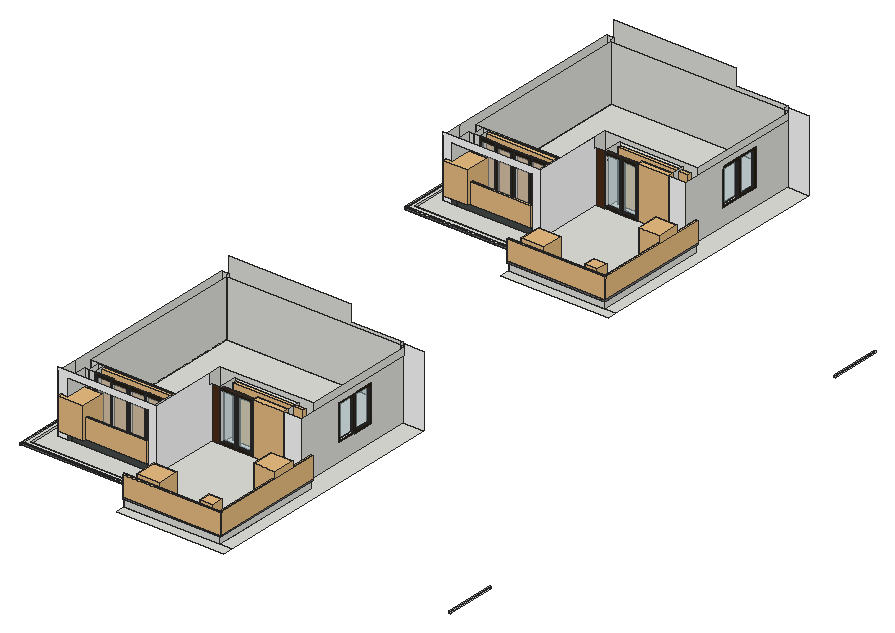
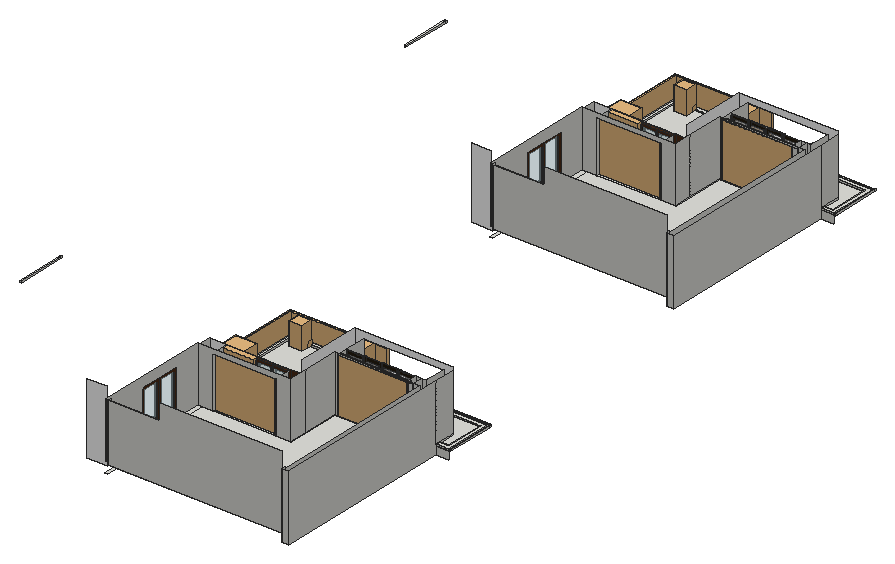
# SketchUp Ruby script. Lengths in inches.
U = 1.inch
M = Sketchup.active_model
def pt(a) = Geom::Point3d.new(a.map { |v| v * U })
def face(e, loops, mat)
  f = e.add_face(loops[0].map { |a| pt(a) })
  loops[1..].each { |l| e.add_face(l.map { |a| pt(a) }).erase! }
  f.material = f.back_material = mat if mat
  f
end
# faces: each face lists its corners as indices into pts; further lists are holes
def faces(e, pts, list, mat = nil) = list.each { |f| face(e, (f[0].is_a?(Array) ? f : [f]).map { |l| l.map { |i| pts[i] } }, mat) }
# xy, xz, yz: faces in a plane at the given z, y or x. An outline is a flat list of corners, or four numbers for a rectangle; further outlines are holes
def ring(l) = l.size == 4 ? [[l[0], l[1]], [l[2], l[1]], [l[2], l[3]], [l[0], l[3]]] : l.each_slice(2).to_a
def flat(e, list, mat, &to3) = list.each { |f| face(e, (f[0].is_a?(Array) ? f : [f]).map { |l| ring(l).map { |u, v| to3.(u, v) } }, mat) }
def xy(e, z, list, mat = nil) = flat(e, list, mat) { |x, y| [x, y, z] }
def xz(e, y, list, mat = nil) = flat(e, list, mat) { |x, z| [x, y, z] }
def yz(e, x, list, mat = nil) = flat(e, list, mat) { |y, z| [x, y, z] }
def lines(e, pts, list) = list.each { |a, b| e.add_line(pt(pts[a]), pt(pts[b])) }
# prism: a flat outline (further loops are holes) pulled along v
def prism(e, loops, v, mat = nil)
  f = face(e, loops, mat); d = Geom::Vector3d.new(v.map { |x| x * U })
  f.pushpull(f.normal.samedirection?(d) ? d.length : -d.length)
end
def box(e, o, s, mat = nil) = prism(e, [[o, [o[0] + s[0], o[1], o[2]], [o[0] + s[0], o[1] + s[1], o[2]], [o[0], o[1] + s[1], o[2]]]], [0, 0, s[2]], mat)
def at(x, y, z, deg = 0) = Geom::Transformation.translation(pt([x, y, z])) * Geom::Transformation.rotation(ORIGIN, Z_AXIS, deg.degrees)
def axes(o, x, y, z) = Geom::Transformation.new([*x, 0, *y, 0, *z, 0, *pt(o).to_a, 1])
def part(name) = M.definitions.add(name)
# library, detail: a bought-in or finely detailed component or shape, given as its bounding box
def library(name, o, s) = part(name).tap { |d| box(d.entities, o, s) }
def detail(e, o, s) = box(e.add_group.entities, o, s)
def put(e, d, t, mat = nil) = e.add_instance(d, t).tap { |i| i.material = mat if mat }
def group(e, t, mat = nil) = e.add_group.tap { |g| g.transformation = t; g.material = mat if mat }.entities
root = M.entities
M.materials.add("[Color M00]").color = [255, 255, 255]
M.materials.add("[Color M05]").color = [114, 114, 114]
M.materials.add("[Slate]").color = [70, 76, 75]
M.materials.add("[Translucent Glass Gray]2").color = [201, 201, 201]
M.materials["[Translucent Glass Gray]2"].alpha = 0.5
M.materials.add("[Translucent Glass Safety]").color = [204, 235, 244]
M.materials["[Translucent Glass Safety]"].alpha = 0.5
M.materials.add("[Wood Veneer 01]").color = [76, 44, 23]
M.materials.add("oak swatch").color = [40, 31, 19]
c1 = library("plant (1)",[-35.72,-28.42,0],[66.31,67.39,84.38])
c2 = library("Glass Railing",[0,0,0],[139.5,4.76,42])
c3 = part("Group\#6")
box(c3.entities,[0,0,0],[1.77,4.72,80.31],"oak swatch")
c4 = part("Exterior Sliding Doors")
xy(c4.entities,0,[[1.77,33.07,3.54,70.87],[1.77,70.87,3.54,108.66]])
xy(c4.entities,0,[[0,0,1.77,33.07],[0,108.66,1.77,141.73]],"oak swatch")
xy(c4.entities,4.72,[[0,4.72,1.77,33.07],[1.77,37.8,3.54,66.14],[1.77,75.88,3.54,103.9375],[0,108.66,1.77,137.01]],"oak swatch")
xy(c4.entities,75.59,[[1.77,37.8,3.54,66.14],[1.77,75.88,3.54,103.9375]])
xy(c4.entities,75.59,[[0,4.72,1.77,33.07],[0,108.66,1.77,137.01]],"oak swatch")
xy(c4.entities,80.31,[[0,0,1.77,33.07],[1.77,33.07,3.54,70.87],[1.77,70.87,3.54,108.66],[0,108.66,1.77,141.73]],"oak swatch")
xz(c4.entities,0,[[0,0,1.77,80.31]],"oak swatch")
xz(c4.entities,4.72,[[0,4.72,1.77,75.59]],"oak swatch")
xz(c4.entities,33.07,[[0,0,1.77,4.72],[1.77,0,3.54,80.31],[0,75.59,1.77,80.31]],"oak swatch")
xz(c4.entities,37.8,[[1.77,4.72,3.54,75.59]])
xz(c4.entities,66.14,[[1.77,4.72,3.54,75.59]],"oak swatch")
xz(c4.entities,70.87,[[1.77,0,3.54,80.31]])
xz(c4.entities,75.88,[[1.77,4.72,3.54,75.59]])
xz(c4.entities,103.9375,[[1.77,4.72,3.54,75.59]],"oak swatch")
xz(c4.entities,108.66,[[1.77,4.72,3.54,75.59]])
xz(c4.entities,108.66,[[0,0,3.54,4.72],[0,75.59,3.54,80.31]],"oak swatch")
xz(c4.entities,137.01,[[0,4.72,1.77,75.59]],"oak swatch")
xz(c4.entities,141.73,[[0,0,1.77,80.31]],"oak swatch")
yz(c4.entities,0,[[0,0,33.07,0,33.07,4.72,4.72,4.72,4.72,75.59,33.07,75.59,33.07,80.31,0,80.31],[108.66,0,141.73,0,141.73,80.31,108.66,80.31,108.66,75.59,137.01,75.59,137.01,4.72,108.66,4.72]],"oak swatch")
yz(c4.entities,1.77,[[4.72,4.72,33.07,75.59],[37.8,4.72,66.14,75.59],[75.88,4.72,103.9375,75.59],[108.66,4.72,137.01,75.59]],"[Translucent Glass Gray]2")
yz(c4.entities,1.77,[[0,0,33.07,0,33.07,4.72,4.72,4.72,4.72,75.59,33.07,75.59,33.07,80.31,0,80.31],[[33.07,0,70.87,80.31],[37.8,4.72,66.14,75.59]],[[70.87,0,141.73,80.31],[108.66,4.72,137.01,75.59],[75.88,4.72,103.9375,75.59]]],"oak swatch")
yz(c4.entities,3.54,[[[33.07,0,70.87,80.31],[37.8,4.72,66.14,75.59]],[[70.87,0,108.66,80.31],[75.88,4.72,103.9375,75.59]]],"oak swatch")
put(c4.entities,c3,at(0,33.07,0))
put(c4.entities,c3,at(0,103.9375,0))
c5 = library("Curtains",[0,0,0],[121.73,8.19,117.22])
c6 = library("Plant",[0,0,0],[12.59,12.59,14.16])
c7 = part("Group\#4")
g1 = group(c7.entities,at(0,0,0))
xy(g1,0,[[0,0,6,48]],"[Wood Veneer 01]")
xy(g1,4,[[0,4,1.8125,44],[1.8125,4,6,44]])
xy(g1,80,[[0,4,1.8125,44],[1.8125,4,6,44]])
xy(g1,84,[[0,0,6,48]],"[Wood Veneer 01]")
xz(g1,0,[[0,0,6,84]],"[Wood Veneer 01]")
xz(g1,4,[[0,4,1.8125,80],[1.8125,4,6,80]])
xz(g1,44,[[0,4,1.8125,80],[1.8125,4,6,80]])
xz(g1,48,[[0,0,6,84]],"[Wood Veneer 01]")
yz(g1,0,[[[0,0,48,84],[4,4,44,80]]],"[Wood Veneer 01]")
yz(g1,1.8125,[[4,4,44,80]],"[Translucent Glass Safety]")
yz(g1,6,[[[0,0,48,84],[4,4,44,80]]],"oak swatch")
g2 = group(c7.entities,at(0,48,0),"oak swatch")
xy(g2,0,[[0,0,6,48]],"[Wood Veneer 01]")
xy(g2,4,[[0,4,1.8125,44],[1.8125,4,6,44]])
xy(g2,80,[[0,4,1.8125,44],[1.8125,4,6,44]])
xy(g2,84,[[0,0,6,48]],"[Wood Veneer 01]")
xz(g2,0,[[0,0,6,84]],"[Wood Veneer 01]")
xz(g2,4,[[0,4,1.8125,80],[1.8125,4,6,80]])
xz(g2,44,[[0,4,1.8125,80],[1.8125,4,6,80]])
xz(g2,48,[[0,0,6,84]],"[Wood Veneer 01]")
yz(g2,0,[[[0,0,48,84],[4,4,44,80]]],"[Wood Veneer 01]")
yz(g2,1.8125,[[4,4,44,80]],"[Translucent Glass Safety]")
yz(g2,6,[[[0,0,48,84],[4,4,44,80]]],"oak swatch")
c8 = library("Flora+17",[-57.52,158.6,-38.64],[66.99,62.88,77.28])
c9 = library("modern+door",[0,0,0],[59.06,11.8125,86.61])
c10 = library("plant1",[-367.84,-375.82,-125.45],[750.59,696.16,1346.74])
c11 = part("skp4FF")
put(c11.entities,c10,at(0,0,0))
xy(root,121.3125,[[491.71,481.81,715.11,502.24],[491.71,502.24,690.8,538.49],[690.8,502.24,715.11,502.24,715.11,1001.66,671.36,1001.66,671.36,738.06,690.8,738.06],[491.71,538.49,690.8,638.99],[279.74,638.99,279.74,1021.31,294.47,1021.31,294.47,662.52,312.05,662.52,312.05,638.99],
  [491.71,638.99,690.8,738.06],[312.05,648.22,312.05,662.52,471.68,662.52,471.68,776.62,481.36,776.62,481.36,648.22],[491.71,738.06,671.36,749.87],[655.66,813.85,662.14,1021.31],[491.71,1481.16,715.11,1501.6],
  [491.71,1501.6,690.8,1537.85],[690.8,1501.6,715.11,1501.6,715.11,2001.02,671.36,2001.02,671.36,1737.41,690.8,1737.41],[491.71,1537.85,690.8,1638.35],[279.74,1638.35,279.74,2020.66,294.47,2020.66,294.47,1661.875,312.05,1661.875,312.05,1638.35],[491.71,1638.35,690.8,1737.41],
  [312.05,1647.57,312.05,1661.875,471.68,1661.875,471.68,1775.97,481.36,1775.97,481.36,1647.57],[491.71,1737.41,671.36,1749.22],[655.66,1813.21,662.14,2020.66]])
xy(root,138.1875,[[491.71,497.56,690.8,502.24],[690.8,497.56,695.49,502.24],[491.71,502.24,491.71,538.49,252.74,538.49,252.74,638.99,279.74,638.99,279.74,630.62,260.99,630.62,260.99,547.12,498.05,547.12,498.05,510.06,684.49,510.06,684.49,724.25,671.36,724.25,671.36,738.06,690.8,738.06,690.8,502.24],[690.8,502.24,695.49,738.06],[498.05,510.06,684.49,510.06,684.49,724.25,671.36,724.25,671.36,738.06,484.3,738.06,484.3,595.06,279.74,595.06,279.74,630.62,260.99,630.62,260.99,547.12,498.05,547.12],
  [249.43,533.81,252.74,538.49],[252.74,533.81,491.71,538.49],[249.43,538.49,252.55,638.99],[252.55,538.49,252.74,638.99],[1142.02,538.49,1145.14,638.99],
  [279.74,595.06,308.96,595.06,308.96,606.41,299.58,606.41,299.58,638.99,279.74,638.99],[466.14,595.06,484.3,638.99],[299.58,606.41,466.14,638.99],[308.96,638.99,321.33,662.52],[321.33,638.99,466.14,662.52],
  [294.47,662.52,471.68,662.52,471.68,776.62,655.66,776.62,655.66,1014.93,294.47,1014.93],[502.34,738.06,634.66,776.62],[655.66,776.62,665.66,1014.93],[294.47,1014.93,655.66,1021.31],[491.71,1496.91,690.8,1501.6],
  [690.8,1496.91,695.49,1501.6],[491.71,1501.6,491.71,1537.85,252.74,1537.85,252.74,1638.35,279.74,1638.35,279.74,1629.97,260.99,1629.97,260.99,1546.47,498.05,1546.47,498.05,1509.41,684.49,1509.41,684.49,1723.61,671.36,1723.61,671.36,1737.41,690.8,1737.41,690.8,1501.6],[690.8,1501.6,695.49,1737.41],[498.05,1509.41,684.49,1509.41,684.49,1723.61,671.36,1723.61,671.36,1737.41,484.3,1737.41,484.3,1594.41,279.74,1594.41,279.74,1629.97,260.99,1629.97,260.99,1546.47,498.05,1546.47],[249.43,1533.16,252.74,1537.85],
  [252.74,1533.16,491.71,1537.85],[1142.02,1533.16,1145.33,1537.85],[249.43,1537.85,252.55,1638.35],[252.55,1537.85,252.74,1638.35],[1142.02,1537.85,1145.14,1638.35],
  [279.74,1594.41,308.96,1594.41,308.96,1605.76,299.58,1605.76,299.58,1638.35,279.74,1638.35],[466.14,1594.41,484.3,1638.35],[299.58,1605.76,466.14,1638.35],[308.96,1638.35,321.33,1661.875],[321.33,1638.35,466.14,1661.875],
  [294.47,1661.875,471.68,1661.875,471.68,1775.97,655.66,1775.97,655.66,2014.29,294.47,2014.29],[502.34,1737.41,634.66,1775.97],[655.66,1775.97,665.66,2014.29],[294.47,2014.29,655.66,2020.66]])
xy(root,141.4375,[[491.71,497.56,695.49,497.56,695.49,738.06,690.8,738.06,690.8,502.24,491.71,502.24],[491.71,502.24,690.8,502.24,690.8,738.06,671.36,738.06,671.36,724.25,684.49,724.25,684.49,510.06,498.05,510.06,498.05,547.12,260.99,547.12,260.99,630.62,279.74,630.62,279.74,638.99,252.74,638.99,252.74,538.49,491.71,538.49],[249.43,533.81,252.74,538.49],[252.74,533.81,491.71,538.49],[249.43,538.49,252.55,638.99],
  [252.55,538.49,252.74,638.99],[1142.02,538.49,1145.14,638.99],[491.71,1496.91,695.49,1496.91,695.49,1737.41,690.8,1737.41,690.8,1501.6,491.71,1501.6],[491.71,1501.6,690.8,1501.6,690.8,1737.41,671.36,1737.41,671.36,1723.61,684.49,1723.61,684.49,1509.41,498.05,1509.41,498.05,1546.47,260.99,1546.47,260.99,1629.97,279.74,1629.97,279.74,1638.35,252.74,1638.35,252.74,1537.85,491.71,1537.85],[249.43,1533.16,252.74,1537.85],
  [252.74,1533.16,491.71,1537.85],[249.43,1537.85,252.55,1638.35],[252.55,1537.85,252.74,1638.35],[1142.02,1537.85,1145.14,1638.35]])
xy(root,152,[[299.58,595.06,308.96,606.41],[308.96,595.06,466.14,606.41],[299.58,1594.41,308.96,1605.76],[308.96,1594.41,466.14,1605.76]],"[Slate]")
xy(root,155.89,[[665.66,833.57,671.36,919.13],[665.66,1832.92,671.36,1918.48]])
xz(root,497.56,[[491.71,138.1875,695.49,141.4375]],"[Color M05]")
xz(root,502.24,[[491.71,121.3125,690.8,138.1875],[491.71,138.1875,690.8,141.4375]])
xz(root,510.06,[[498.05,138.1875,684.49,141.4375]])
xz(root,533.81,[[249.43,138.1875,252.74,141.4375],[1142.02,138.1875,1145.33,141.4375]])
xz(root,533.81,[[252.74,138.1875,491.71,141.4375]],"[Color M05]")
xz(root,538.49,[[249.43,138.1875,252.55,141.4375],[252.55,138.1875,252.74,141.4375],[252.74,138.1875,491.71,141.4375],[1142.02,138.1875,1145.14,141.4375]])
xz(root,547.12,[[260.99,138.1875,498.05,141.4375]])
xz(root,595.06,[[279.74,138.1875,299.58,138.1875,299.58,252.5,466.14,252.5,466.14,138.1875,484.3,138.1875,484.3,265.6875,279.74,265.6875]],"[Color M00]")
xz(root,595.06,[[299.58,138.1875,308.96,152],[308.96,138.1875,466.14,152]],"[Slate]")
xz(root,606.41,[[299.58,138.1875,308.96,152],[308.96,138.1875,466.14,152]])
xz(root,630.62,[[260.99,138.1875,279.74,141.4375]])
xz(root,638.99,[[252.74,121.3125,279.74,138.1875],[249.43,138.1875,252.55,141.4375],[252.55,138.1875,252.74,141.4375],[252.74,138.1875,279.74,141.4375],[299.58,138.1875,308.96,252.5],
  [308.96,138.1875,321.33,252.5],[1142.02,138.1875,1145.14,141.4375]])
xz(root,662.52,[[294.47,121.3125,471.68,138.1875],[294.47,138.1875,294.47,254.625,471.68,254.625,471.68,138.1875,466.14,138.1875,466.14,252.5,308.96,252.5,308.96,138.1875],[308.96,138.1875,321.33,252.5]])
xz(root,724.25,[[671.36,138.1875,684.49,141.4375]])
xz(root,738.06,[[671.36,121.3125,690.8,138.1875],[671.36,138.1875,690.8,141.4375],[690.8,138.1875,695.49,141.4375]])
xz(root,738.06,[[634.66,138.1875,671.36,244.75]],"[Color M00]")
xz(root,738.06,[[484.3,138.1875,502.34,244.75]],"[Wood Veneer 01]")
xz(root,776.62,[[471.68,138.1875,471.68,254.625,665.66,254.625,665.66,138.1875,634.66,138.1875,634.66,244.75,502.34,244.75,502.34,138.1875]])
xz(root,833.57,[[665.66,155.89,671.36,232.14]])
xz(root,919.13,[[665.66,155.89,671.36,232.14]])
xz(root,1001.66,[[671.36,121.3125,715.11,121.3125,715.11,269.375,674.49,269.375,674.49,244.75,671.36,244.75]],"[Color M00]")
xz(root,1014.93,[[294.47,138.1875,655.66,254.625],[655.66,138.1875,665.66,254.625]])
xz(root,1021.31,[[279.74,121.3125,294.47,258.1875],[294.47,138.1875,294.47,291.125,548.11,291.125,548.11,258.1875,655.66,258.1875,655.66,138.1875]])
xz(root,1496.91,[[491.71,138.1875,695.49,141.4375]],"[Color M05]")
xz(root,1501.6,[[491.71,121.3125,690.8,138.1875],[491.71,138.1875,690.8,141.4375]])
xz(root,1509.41,[[498.05,138.1875,684.49,141.4375]])
xz(root,1533.16,[[249.43,138.1875,252.74,141.4375],[1142.02,138.1875,1145.33,141.4375]])
xz(root,1533.16,[[252.74,138.1875,491.71,141.4375]],"[Color M05]")
xz(root,1537.85,[[249.43,138.1875,252.55,141.4375],[252.55,138.1875,252.74,141.4375],[252.74,138.1875,491.71,141.4375],[1142.02,138.1875,1145.14,141.4375]])
xz(root,1546.47,[[260.99,138.1875,498.05,141.4375]])
xz(root,1594.41,[[279.74,138.1875,299.58,138.1875,299.58,252.5,466.14,252.5,466.14,138.1875,484.3,138.1875,484.3,265.6875,279.74,265.6875]],"[Color M00]")
xz(root,1594.41,[[299.58,138.1875,308.96,152],[308.96,138.1875,466.14,152]],"[Slate]")
xz(root,1605.76,[[299.58,138.1875,308.96,152],[308.96,138.1875,466.14,152]])
xz(root,1629.97,[[260.99,138.1875,279.74,141.4375]])
xz(root,1638.35,[[252.74,121.3125,279.74,138.1875],[249.43,138.1875,252.55,141.4375],[252.55,138.1875,252.74,141.4375],[252.74,138.1875,279.74,141.4375],[299.58,138.1875,308.96,252.5],
  [308.96,138.1875,321.33,252.5],[1142.02,138.1875,1145.14,141.4375]])
xz(root,1661.875,[[294.47,121.3125,471.68,138.1875],[294.47,138.1875,294.47,254.625,471.68,254.625,471.68,138.1875,466.14,138.1875,466.14,252.5,308.96,252.5,308.96,138.1875],[308.96,138.1875,321.33,252.5]])
xz(root,1723.61,[[671.36,138.1875,684.49,141.4375]])
xz(root,1737.41,[[671.36,121.3125,690.8,138.1875],[671.36,138.1875,690.8,141.4375],[690.8,138.1875,695.49,141.4375]])
xz(root,1737.41,[[634.66,138.1875,671.36,244.75]],"[Color M00]")
xz(root,1737.41,[[484.3,138.1875,502.34,244.75]],"[Wood Veneer 01]")
xz(root,1775.97,[[471.68,138.1875,471.68,254.625,665.66,254.625,665.66,138.1875,634.66,138.1875,634.66,244.75,502.34,244.75,502.34,138.1875]])
xz(root,1832.92,[[665.66,155.89,671.36,232.14]])
xz(root,1918.48,[[665.66,155.89,671.36,232.14]])
xz(root,2001.02,[[671.36,121.3125,715.11,121.3125,715.11,269.375,674.49,269.375,674.49,244.75,671.36,244.75]],"[Color M00]")
xz(root,2014.29,[[294.47,138.1875,655.66,254.625],[655.66,138.1875,665.66,254.625]])
xz(root,2020.66,[[279.74,121.3125,294.47,258.1875],[294.47,138.1875,294.47,291.125,548.11,291.125,548.11,258.1875,655.66,258.1875,655.66,138.1875]])
yz(root,249.43,[[533.81,138.1875,538.49,141.4375],[538.49,138.1875,638.99,141.4375],[1533.16,138.1875,1537.85,141.4375],[1537.85,138.1875,1638.35,141.4375]])
yz(root,252.55,[[538.49,138.1875,638.99,141.4375],[1537.85,138.1875,1638.35,141.4375]])
yz(root,252.74,[[533.81,138.1875,538.49,141.4375],[538.49,138.1875,638.99,141.4375],[1533.16,138.1875,1537.85,141.4375],[1537.85,138.1875,1638.35,141.4375]])
yz(root,260.99,[[547.12,138.1875,630.62,141.4375],[1546.47,138.1875,1629.97,141.4375]])
yz(root,279.74,[[638.99,121.3125,1021.31,258.1875],[1638.35,121.3125,2020.66,258.1875],[595.06,138.1875,630.62,141.4375],[630.62,138.1875,638.99,141.4375],[1594.41,138.1875,1629.97,141.4375],
  [1629.97,138.1875,1638.35,141.4375],[595.06,141.4375,638.99,258.1875],[1594.41,141.4375,1638.35,258.1875]])
yz(root,294.47,[[662.52,121.3125,1021.31,138.1875],[1661.875,121.3125,2020.66,138.1875],[662.52,138.1875,1014.93,254.625],[1014.93,138.1875,1021.31,258.1875],[1661.875,138.1875,2014.29,254.625],
  [2014.29,138.1875,2020.66,258.1875]])
yz(root,299.58,[[606.41,138.1875,638.99,138.1875,638.99,252.5,595.06,252.5,595.06,152,606.41,152],[1605.76,138.1875,1638.35,138.1875,1638.35,252.5,1594.41,252.5,1594.41,152,1605.76,152]])
yz(root,308.96,[[595.06,138.1875,606.41,152],[638.99,138.1875,662.52,252.5],[1594.41,138.1875,1605.76,152],[1638.35,138.1875,1661.875,252.5]])
yz(root,321.33,[[638.99,138.1875,662.52,252.5],[1638.35,138.1875,1661.875,252.5]])
yz(root,466.14,[[595.06,138.1875,606.41,152],[606.41,138.1875,606.41,152,595.06,152,595.06,252.5,638.99,252.5,638.99,138.1875],[638.99,138.1875,662.52,252.5],[1594.41,138.1875,1605.76,152],[1605.76,138.1875,1605.76,152,1594.41,152,1594.41,252.5,1638.35,252.5,1638.35,138.1875],
  [1638.35,138.1875,1661.875,252.5]])
yz(root,471.68,[[662.52,121.3125,738.06,138.1875],[738.06,121.3125,776.62,138.1875],[1661.875,121.3125,1737.41,138.1875],[1737.41,121.3125,1775.97,138.1875],[662.52,138.1875,738.06,254.625],
  [738.06,138.1875,776.62,254.625],[1661.875,138.1875,1737.41,254.625],[1737.41,138.1875,1775.97,254.625]])
yz(root,484.3,[[595.06,138.1875,738.06,138.1875,738.06,244.75,731.24,244.75,731.24,265.6875,595.06,265.6875],[1594.41,138.1875,1737.41,138.1875,1737.41,244.75,1730.6,244.75,1730.6,265.6875,1594.41,265.6875]],"[Color M00]")
yz(root,491.71,[[502.24,121.3125,538.49,138.1875],[1501.6,121.3125,1537.85,138.1875],[497.56,138.1875,502.24,141.4375],[502.24,138.1875,533.81,141.4375],[533.81,138.1875,538.49,141.4375],
  [1496.91,138.1875,1501.6,141.4375],[1501.6,138.1875,1533.16,141.4375],[1533.16,138.1875,1537.85,141.4375]])
yz(root,498.05,[[510.06,138.1875,547.12,141.4375],[1509.41,138.1875,1546.47,141.4375]])
yz(root,502.34,[[738.06,138.1875,776.62,244.75],[1737.41,138.1875,1775.97,244.75]])
yz(root,634.66,[[738.06,138.1875,776.62,244.75],[1737.41,138.1875,1775.97,244.75]])
yz(root,655.66,[[1014.93,138.1875,1021.31,258.1875],[2014.29,138.1875,2020.66,258.1875]])
yz(root,665.66,[[[776.62,138.1875,1014.93,254.625],[833.57,155.89,919.13,232.14]],[[1775.97,138.1875,2014.29,254.625],[1832.92,155.89,1918.48,232.14]]])
yz(root,671.36,[[[738.06,121.3125,1001.66,244.75],[833.57,155.89,919.13,232.14]],[[1737.41,121.3125,2001.02,244.75],[1832.92,155.89,1918.48,232.14]],[724.25,138.1875,738.06,141.4375],[1723.61,138.1875,1737.41,141.4375]])
yz(root,684.49,[[510.06,138.1875,724.25,141.4375],[1509.41,138.1875,1723.61,141.4375]])
yz(root,690.8,[[502.24,121.3125,738.06,138.1875],[1501.6,121.3125,1737.41,138.1875],[502.24,138.1875,738.06,141.4375],[1501.6,138.1875,1737.41,141.4375]])
yz(root,695.49,[[497.56,138.1875,738.06,141.4375],[1496.91,138.1875,1737.41,141.4375]],"[Color M05]")
yz(root,1142.02,[[533.81,138.1875,538.49,141.4375],[538.49,138.1875,638.99,141.4375],[1533.16,138.1875,1537.85,141.4375],[1537.85,138.1875,1638.35,141.4375]])
put(root,c1,axes([314.87,1607.49,153.49],[0.77,0,0],[0,0.77,0],[0,0,0.77]))
put(root,c1,axes([314.87,608.13,153.49],[0.77,0,0],[0,0.77,0],[0,0,0.77]))
put(root,c2,axes([299.58,1591.4375,152.79],[1.194,0,0],[0,1,0],[0,0,1]))
put(root,c2,axes([299.58,592.08,152.79],[1.194,0,0],[0,1,0],[0,0,1]))
put(root,c4,axes([322.3125,1640.12,138.1875],[0,-1,0],[0.99858,0,0],[0,0,1.4151]))
put(root,c4,axes([322.3125,640.77,138.1875],[0,-1,0],[0.99858,0,0],[0,0,1.4151]))
put(root,c5,axes([320.79,1653.68,138.1875],[1.19408,0,0],[0,1,0],[0,0,0.96546]))
put(root,c5,axes([320.79,654.32,138.1875],[1.19408,0,0],[0,1,0],[0,0,0.96546]))
put(root,c6,axes([508.4,1517.43,138.1875],[0.7,0,0],[0,0.7,0],[0,0,0.7]))
put(root,c6,axes([508.4,518.07,138.1875],[0.7,0,0],[0,0.7,0],[0,0,0.7]))
put(root,c7,axes([501.82,1743.41,138.1875],[0,-1,0],[0.71,0,0],[0,0,1.26]))
put(root,c7,axes([501.82,744.06,138.1875],[0,-1,0],[0.71,0,0],[0,0,1.26]))
put(root,c8,axes([554.58,1393.6875,160.89],[0.71,0,0],[0,0.71,0],[0,0,0.71]))
put(root,c8,axes([554.58,394.33,160.89],[0.71,0,0],[0,0.71,0],[0,0,0.71]))
put(root,c5,axes([509.39,1761.9,130.52],[1.19408,0,0],[0,1,0],[0,0,0.96546]))
put(root,c5,axes([509.39,762.55,130.52],[1.19408,0,0],[0,1,0],[0,0,0.96546]))
put(root,c2,axes([491.82,1496.91,141.4375],[1.46,0,0],[0,1,0],[0,0,1]))
put(root,c2,axes([491.82,497.56,141.4375],[1.46,0,0],[0,1,0],[0,0,1]))
put(root,c9,axes([570.29,1737.41,138.1875],[1.09,0,0],[0,1,0],[0,0,1.23031]))
put(root,c9,axes([570.29,738.06,138.1875],[1.09,0,0],[0,1,0],[0,0,1.23031]))
put(root,c6,axes([644.35,1505.95,138.1875],[0.7,0,0],[0,0.7,0],[0,0,0.7]))
put(root,c6,axes([644.35,506.59,138.1875],[0.7,0,0],[0,0.7,0],[0,0,0.7]))
put(root,c11,axes([657.83,1519.74,142.62],[0.03534,0,0],[0,0.03534,0],[0,0,0.03534]))
put(root,c11,axes([657.83,520.38,142.62],[0.03534,0,0],[0,0.03534,0],[0,0,0.03534]))
put(root,c7,axes([665.36,1832.92,155.89],[1,0,0],[0,0.88868,0],[0,0,0.90774]))
put(root,c7,axes([665.36,833.57,155.89],[1,0,0],[0,0.88868,0],[0,0,0.90774]))
put(root,c1,axes([675,1658.45,141.4375],[0.67,0,0],[0,0.67,0],[0,0,0.67]))
put(root,c1,axes([675,659.09,141.4375],[0.67,0,0],[0,0.67,0],[0,0,0.67]))
put(root,c2,axes([695.56,1499.92,141.41],[0,1.70244,0],[-1,0,0],[0,0,1]))
put(root,c2,axes([695.56,500.57,141.41],[0,1.70244,0],[-1,0,0],[0,0,1]))
